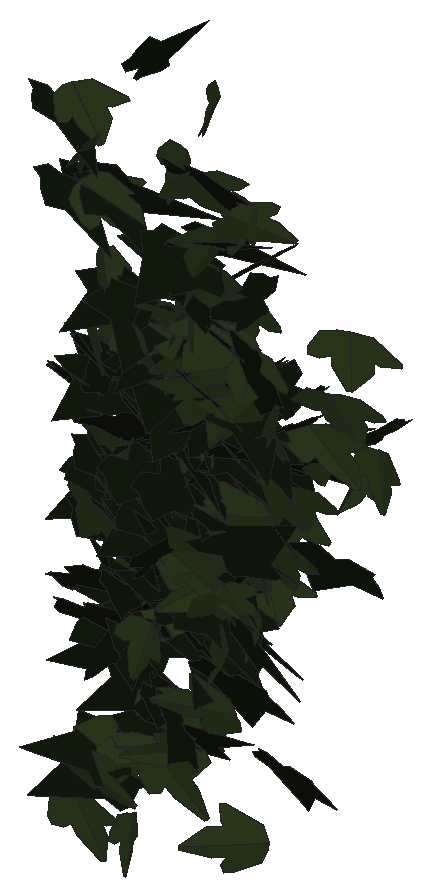
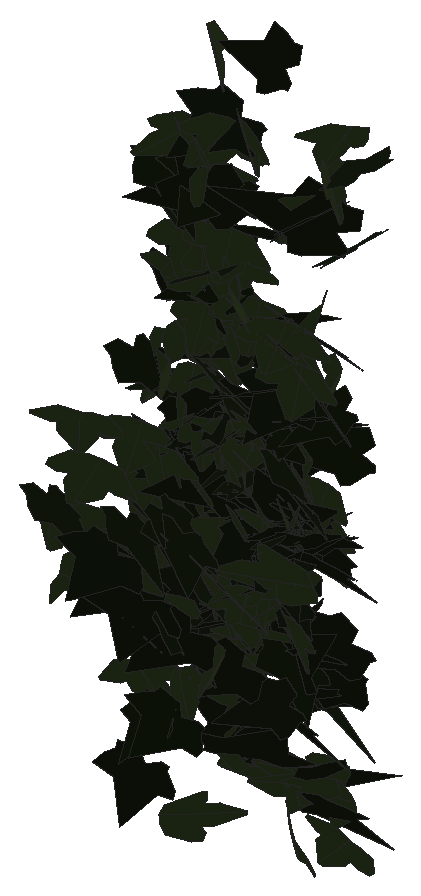
# SketchUp Ruby script. Lengths in millimetres.
U = 1.mm
M = Sketchup.active_model
def pt(a) = Geom::Point3d.new(a.map { |v| v * U })
def face(e, loops, mat)
  f = e.add_face(loops[0].map { |a| pt(a) })
  loops[1..].each { |l| e.add_face(l.map { |a| pt(a) }).erase! }
  f.material = f.back_material = mat if mat
  f
end
# faces: each face lists its corners as indices into pts; further lists are holes
def faces(e, pts, list, mat = nil) = list.each { |f| face(e, (f[0].is_a?(Array) ? f : [f]).map { |l| l.map { |i| pts[i] } }, mat) }
# xy, xz, yz: faces in a plane at the given z, y or x. An outline is a flat list of corners, or four numbers for a rectangle; further outlines are holes
def ring(l) = l.size == 4 ? [[l[0], l[1]], [l[2], l[1]], [l[2], l[3]], [l[0], l[3]]] : l.each_slice(2).to_a
def flat(e, list, mat, &to3) = list.each { |f| face(e, (f[0].is_a?(Array) ? f : [f]).map { |l| ring(l).map { |u, v| to3.(u, v) } }, mat) }
def xy(e, z, list, mat = nil) = flat(e, list, mat) { |x, y| [x, y, z] }
def xz(e, y, list, mat = nil) = flat(e, list, mat) { |x, z| [x, y, z] }
def yz(e, x, list, mat = nil) = flat(e, list, mat) { |y, z| [x, y, z] }
def lines(e, pts, list) = list.each { |a, b| e.add_line(pt(pts[a]), pt(pts[b])) }
# prism: a flat outline (further loops are holes) pulled along v
def prism(e, loops, v, mat = nil)
  f = face(e, loops, mat); d = Geom::Vector3d.new(v.map { |x| x * U })
  f.pushpull(f.normal.samedirection?(d) ? d.length : -d.length)
end
def box(e, o, s, mat = nil) = prism(e, [[o, [o[0] + s[0], o[1], o[2]], [o[0] + s[0], o[1] + s[1], o[2]], [o[0], o[1] + s[1], o[2]]]], [0, 0, s[2]], mat)
def at(x, y, z, deg = 0) = Geom::Transformation.translation(pt([x, y, z])) * Geom::Transformation.rotation(ORIGIN, Z_AXIS, deg.degrees)
def axes(o, x, y, z) = Geom::Transformation.new([*x, 0, *y, 0, *z, 0, *pt(o).to_a, 1])
def part(name) = M.definitions.add(name)
# library, detail: a bought-in or finely detailed component or shape, given as its bounding box
def library(name, o, s) = part(name).tap { |d| box(d.entities, o, s) }
def detail(e, o, s) = box(e.add_group.entities, o, s)
def put(e, d, t, mat = nil) = e.add_instance(d, t).tap { |i| i.material = mat if mat }
def group(e, t, mat = nil) = e.add_group.tap { |g| g.transformation = t; g.material = mat if mat }.entities
root = M.entities
M.materials.add("efeu1").color = [18, 25, 13]
M.materials.add("efeu2").color = [43, 57, 29]
c1 = part("ivyleaf_9")
p = [[39.1,54.8,31.7],[34.5,51.8,30.2],[-5.3,25.2,17.3],[-17.9,28.3,20.9],[-21.6,21.7,17],[-20.2,4.3,5.3],
  [-22.9,-0.3,2.5],[-17.1,-4,-0.6],[-2,-2.1,-1.2],[-0.7,-15.4,-10.1],[16.6,-22.3,-16.7],[21.1,-15.1,-12.5],
  [32.7,-10.7,-11],[46.1,-1.8,-6.6],[30.8,11.2,3.8]]
faces(c1.entities,p,[[0,1,2,3,4,5,6,7,8,9,10,11,12,13,14]],"efeu1")
c2 = part("ivyleaf_10")
p = [[0,12.8,-0.8],[-1.5,51.3,-10.9],[-4.9,51,-11.6],[-13.6,26.5,-7.3],[-13.2,15.9,-4.6],[-21.1,19.3,-7.2],
  [-29.5,16.3,-8.3],[-29.2,8.3,-6.2],[-19.7,-9.8,0.5],[-7.6,-13,4],[1,-12.2,5.8],[-0.4,51.1,-11.1],
  [-1.5,51.1,-10.9],[1,-12.4,5.9],[16.9,-12.4,3.5],[35.1,9.1,-5.1],[35,12.9,-6.1],[20.5,16.4,-4.9],
  [15.8,15,-3.8],[15.3,27.6,-7.1],[12.8,31.3,-7.8]]
faces(c2.entities,p,[[0,1,2,3,4,5,6,7,8,9,10],[11,12,0,13,14,15,16,17,18,19,20]],"efeu2")
put(root,c1,axes([3673.6,933.8,2008.3],[-1.71532,0.04055,0.01997],[-0.04734,-0.11203,-0.89509],[-0.07184,-0.89452,0.11301]))
put(root,c1,axes([3633.8,892.5,2375.7],[0.49599,-0.92629,-0.17661],[-0.02252,0.18,-0.96155],[1.79453,0.25827,0.03674]))
put(root,c1,axes([3632.3,890.9,2463.7],[0.18435,-0.94135,0.27937],[0.2943,-0.26259,-0.93845],[1.84548,0.13591,0.12175]))
put(root,c1,axes([3621.6,907.3,2137],[1.51771,-0.42905,0.25621],[0.48544,-0.06545,-0.9035],[0.81787,0.83504,0.06083]))
put(root,c2,axes([3662.9,917.6,2079.5],[-1.57272,0.45852,0.04383],[-0.08821,0.00679,-0.9449],[-0.87218,-0.82749,0.01653]))
put(root,c1,axes([3685.3,905.5,1840.2],[-1.14241,0.84092,0.03289],[-0.03684,0.02659,-1.03317],[-1.60123,-0.60057,0.00031]))
put(root,c1,axes([3635.1,909.2,1905.6],[1.52663,0.25674,0.39294],[0.70805,0.12662,-0.8422],[-0.54468,0.88419,0.00651]))
put(root,c2,axes([3659.8,1097.4,1962.1],[-0.8183,0.80707,0.14351],[-0.0896,0.13748,-0.91417],[-1.55754,-0.43193,-0.02281]))
put(root,c1,axes([3647.9,912.1,1868.8],[1.7241,0.26652,-0.11191],[-0.20646,-0.02779,-0.94428],[-0.50994,0.91236,0.00393]))
put(root,c1,axes([3642.4,908.2,2180.9],[1.4894,-0.46447,-0.25853],[-0.34559,0.19885,-0.90691],[0.95083,0.79983,0.07534]))
put(root,c1,axes([3686.7,906.5,1696.9],[-1.77573,-0.06272,0.18686],[-0.35243,-0.03072,-0.93496],[0.12848,-0.95105,0.01788]))
put(root,c1,axes([3688.4,1086.8,2056.5],[-1.34517,0.55722,0.10387],[-0.13983,0.07455,-0.89993],[-1.06966,-0.71048,-0.01297]))
put(root,c1,axes([3688.9,901.6,1719.6],[-0.82429,-0.21345,0.80804],[-1.3079,-0.42699,-0.48113],[0.90523,-0.81129,0.04063]))
put(root,c2,axes([3681.3,880.4,2011],[-1.3261,0.43299,0.38568],[-0.75303,0.08574,-0.81106],[-0.80674,-0.79177,0.12309]))
put(root,c2,axes([3661.1,897.6,2214.7],[-0.71641,0.86082,-0.25507],[0.11633,-0.25136,-0.93854],[-1.70476,-0.37891,0.04314]))
put(root,c1,axes([3651.4,930,2047.7],[0.24151,-0.91044,-0.05985],[-0.03003,0.05823,-0.91921],[1.73623,0.12765,-0.00757]))
put(root,c1,axes([3656.9,932.6,2023.4],[-0.24965,-0.9069,0.01351],[0.00625,-0.01413,-0.91633],[1.7262,-0.13111,0.00527]))
put(root,c1,axes([3680.8,942.3,1886.8],[0.11527,0.89691,-0.00348],[0.00089,-0.00352,-0.89895],[-1.70701,0.06057,-0.00071]))
put(root,c2,axes([3673.5,953.1,1932.2],[1.08008,-0.65356,-0.19834],[-0.1506,0.19322,-0.86311],[1.29112,0.56927,0.06525]))
put(root,c1,axes([3671.3,935.7,2031.8],[-0.96682,-0.73449,-0.17827],[0.20746,0.14135,-0.893],[1.42342,-0.51948,0.00907]))
put(root,c2,axes([3652,889.4,1649.2],[1.47018,-0.15436,0.51226],[0.98157,-0.02442,-0.78509],[0.27078,0.92657,0.06465]))
put(root,c2,axes([3680,880.1,2443.5],[0.12874,-0.98974,-0.17322],[-0.00011,0.17361,-0.99198],[1.91231,0.06664,0.01161]))
put(root,c1,axes([3700.6,883.6,2176.2],[-0.37681,0.67605,0.75201],[-0.40511,0.72125,-0.70444],[-1.88143,-0.2907,0.00107]))
put(root,c2,axes([3675.4,943.3,1979.2],[0.6443,0.79194,-0.24251],[-0.28138,-0.19999,-0.85949],[-1.55099,0.36526,0.05519]))
put(root,c2,axes([3666.6,875.2,2492.4],[0.80908,0.86432,0.23318],[0.15964,0.21854,-0.96299],[-1.69629,0.43282,0.02059]))
put(root,c2,axes([3692.5,913.5,2111.1],[0.7486,-0.38137,0.77451],[-1.07561,0.52963,0.54781],[-1.24205,-0.68852,-0.0076]))
put(root,c1,axes([3692.1,908.3,2150.2],[-1.39319,-0.49642,0.31362],[-0.37268,-0.26614,-0.87834],[1.05356,-0.75059,0.10402]))
put(root,c1,axes([3653.6,989.4,1859.6],[1.57955,-0.29876,0.07791],[0.14587,-0.0171,-0.88203],[0.56922,0.83342,0.00983]))
put(root,c1,axes([3701.1,936.6,1868.7],[0.44897,-0.56937,0.88839],[-0.70102,0.80863,0.61605],[-1.88191,-0.43705,-0.01754]))
put(root,c1,axes([3673.8,1143.5,1905.5],[0.93234,0.63225,0.44227],[0.43948,0.37974,-0.79862],[-1.40117,0.5398,0.04379]))
put(root,c2,axes([3678.9,903.4,2290.8],[-0.04781,0.92926,-0.26709],[-0.02416,-0.26748,-0.9294],[-1.84001,-0.02063,0.01914]))
put(root,c2,axes([3660.3,890.3,1702.9],[-0.55459,0.19597,-0.84689],[1.32875,-0.47938,-0.35115],[-0.98562,-0.75653,0.00313]))
put(root,c1,axes([3678.8,946,1845.8],[-0.77992,-0.92763,-0.36512],[0.27358,0.33565,-1.01411],[1.87747,-0.43426,-0.0039]))
put(root,c1,axes([3688.7,941.2,1891],[-1.20376,-0.62089,-0.15637],[0.30026,0.0619,-0.8839],[1.181,-0.64859,0.06534]))
put(root,c2,axes([3689.4,920.3,2060.8],[-0.55356,0.87086,-0.01631],[-0.19104,-0.0506,-0.91139],[-1.64667,-0.28689,0.11122]))
put(root,c2,axes([3697.3,915,2208.3],[-1.77322,0.17086,0.08642],[-0.1535,0.03915,-0.94694],[-0.33051,-0.93488,-0.02386]))
put(root,c1,axes([3712.1,920.9,2097.4],[-0.69109,0.85796,0.0877],[-0.04289,0.08569,-0.93156],[-1.64082,-0.3636,-0.01259]))
put(root,c1,axes([3709.3,905.8,2263.1],[-1.7922,0.09839,-0.16926],[0.27296,-0.21934,-0.92542],[-0.25364,-0.93129,0.20007]))
put(root,c1,axes([3705.4,931.4,1979.3],[-0.19569,0.86544,-0.20515],[0.09309,-0.2007,-0.87119],[-1.69019,-0.11125,-0.02423]))
put(root,c2,axes([3697.7,909.9,2084.3],[0.8017,-0.84181,-0.02418],[-0.01234,0.02379,-0.94131],[1.60275,0.42126,0.00485]))
put(root,c1,axes([3683.5,911.3,1919.9],[0.95433,-0.62284,-0.48454],[-0.53446,0.39567,-0.79921],[1.40353,0.57417,0.02513]))
put(root,c1,axes([3719,919.2,1802.1],[-1.59107,0.31556,-0.01671],[0.0298,-0.00583,-0.89357],[-0.60067,-0.83614,-0.00008]))
put(root,c2,axes([3700.4,1102.4,1922.8],[-0.13731,-0.91445,-0.08181],[0.09265,0.07814,-0.91632],[1.74487,-0.07611,0.04222]))
put(root,c1,axes([3692.5,932.5,2049.3],[-1.24832,0.08888,0.63468],[1.19641,-0.08744,0.6619],[0.23727,0.90851,0.00162]))
put(root,c2,axes([3700.6,915.8,2072.8],[-1.41826,0.5426,-0.01916],[0.03178,-0.00962,-0.92181],[-1.03283,-0.74538,-0.00205]))
put(root,c2,axes([3670.4,895.9,1725.2],[0.28044,0.12175,-1.01603],[1.67002,0.51309,0.18874],[1.00198,-0.88925,-0.03021]))
put(root,c2,axes([3700.4,927.6,2061.9],[0.8884,-0.78576,0.08376],[0.08647,-0.07043,-0.91395],[1.50144,0.46899,0.00308]))
put(root,c1,axes([3684,909.6,1997.7],[1.30839,-0.54835,-0.26594],[-0.33255,0.20672,-0.87793],[1.11119,0.70753,0.0504]))
put(root,c1,axes([3713.6,1086.4,2085.7],[0.28701,0.86465,0.2661],[-0.11277,0.27864,-0.87179],[-1.71807,0.12615,0.10167]))
put(root,c1,axes([3692.4,935.4,2035.8],[-0.25078,-0.86286,-0.26158],[0.03165,0.26199,-0.87258],[1.7157,-0.13095,-0.02214]))
put(root,c2,axes([3707.8,928.1,2062.4],[0.49554,-0.88612,0.04843],[0.03813,-0.04459,-0.92355],[1.68854,0.26105,0.00664]))
put(root,c1,axes([3673.9,934.2,1954.5],[1.20184,-0.53306,0.33993],[0.58025,-0.16414,-0.82376],[1.05409,0.69813,0.06588]))
put(root,c2,axes([3667.5,958.7,1989.3],[0.44823,0.13556,1.03923],[1.80336,0.42759,-0.27051],[-0.8523,0.97603,-0.02583]))
put(root,c1,axes([3690.5,944.4,1953.2],[0.35667,-0.87156,-0.08214],[-0.00877,0.08302,-0.89138],[1.66607,0.18702,0.01289]))
put(root,c2,axes([3704.3,945.6,1962],[-0.67994,-0.81536,-0.11006],[0.4707,0.00801,-0.86217],[1.49345,-0.37374,0.22162]))
put(root,c2,axes([3691.9,869.8,2390],[0.61478,0.79126,0.65933],[0.49777,0.60533,-0.85459],[-1.89596,0.4155,-0.01057]))
put(root,c2,axes([3741.5,879.5,2220.3],[-0.65799,0.15548,0.96307],[-1.72579,0.32558,-0.37808],[-0.68468,-0.97007,0.02747]))
put(root,c1,axes([3685.7,895.9,2004.7],[-0.68785,-0.14762,-0.92172],[1.65761,0.30226,-0.38992],[0.63915,-0.94277,0.01931]))
put(root,c1,axes([3692.2,890.4,2390.5],[0.35411,-0.92804,-0.29168],[-0.01544,0.29547,-0.9453],[1.85137,0.17997,0.04791]))
put(root,c1,axes([3706.3,886.2,2124.4],[1.58719,0.60909,-0.12871],[-0.19721,-0.07635,-1.0327],[-1.16829,0.84037,-0.00053]))
put(root,c1,axes([3708,1135.4,1899.4],[1.34652,-0.15041,-0.56051],[-0.92493,0.3295,-0.70186],[0.60367,0.84034,0.17488]))
put(root,c1,axes([3688.2,920.3,2049.2],[0.84329,-0.86355,0.20883],[0.16488,-0.19025,-0.97055],[1.68283,0.45138,-0.00955]))
put(root,c2,axes([3693,899,1710.6],[0.23826,0.06353,-0.9519],[1.24569,0.69275,0.13232],[1.32097,-0.66474,0.04691]))
put(root,c1,axes([3729.9,1087.7,1979.2],[-0.89479,0.7237,-0.34333],[0.39298,-0.27515,-0.86274],[-1.47296,-0.51304,-0.02161]))
put(root,c1,axes([3671.2,891,2381.4],[1.00697,-0.12814,0.96083],[1.7784,-0.22372,-0.54439],[0.49067,1.07382,0.00124]))
put(root,c1,axes([3697.8,939.4,2030],[0.79982,-0.79543,-0.09642],[0.00516,0.1103,-0.89803],[1.52494,0.41683,0.05362]))
put(root,c2,axes([3705.9,904.7,1640.8],[0.97007,-0.55797,0.59763],[0.73939,-0.45439,-0.75557],[1.36919,0.6407,-0.0154]))
put(root,c1,axes([3703.8,1091.7,1974.6],[1.71986,0.21326,-0.00118],[0.00926,-0.02576,-0.92812],[-0.40578,0.9033,-0.02619]))
put(root,c2,axes([3721.4,910.3,2248.9],[-1.62044,-0.39436,-0.18271],[0.37818,0.0042,-0.93506],[0.73568,-0.8708,0.07823]))
put(root,c2,axes([3720.5,939.2,1911.9],[-0.34348,0.75935,-0.45575],[-0.04259,-0.46888,-0.77236],[-1.68497,-0.14294,0.11243]))
put(root,c1,axes([3740.8,1081.4,2101.7],[-0.80414,0.70772,-0.39931],[0.23909,-0.38777,-0.82018],[-1.52795,-0.43314,0.08181]))
put(root,c1,axes([3718.6,899.4,2176],[1.77263,-0.09802,-0.35514],[-0.67049,0.04552,-0.93651],[0.20514,0.99577,0.00785]))
put(root,c1,axes([3727.5,936.7,2052],[-1.29476,-0.41985,-0.43111],[0.78244,0.15088,-0.79571],[0.83633,-0.79114,0.07703]))
put(root,c2,axes([3724.2,942.7,1898.7],[1.51901,0.41228,0.0331],[0.066,0.00498,-0.89826],[-0.78441,0.79881,-0.01148]))
put(root,c1,axes([3712.3,993.7,1887.9],[1.69486,0.04618,0.03504],[0.06595,0.00842,-0.8917],[-0.08845,0.89118,0.00661]))
put(root,c1,axes([3754.4,937.2,1743.8],[-1.91641,-0.35404,0.19197],[0.36027,0.04022,1.06708],[-0.67654,1.02429,0.02446]))
put(root,c1,axes([3733.7,899.8,2257.4],[-0.97642,-0.81769,0.05598],[-0.00397,-0.06474,-0.96476],[1.55986,-0.51201,0.03259]))
put(root,c1,axes([3744.7,902.6,1999],[-1.11286,-0.44155,0.53269],[-0.39793,-0.55207,-0.68712],[1.25526,-0.56647,0.25443]))
put(root,c2,axes([3726.6,931.8,2024],[1.6998,-0.04927,0.11951],[0.23185,0.04166,-0.8932],[0.0823,0.90012,0.04788]))
put(root,c1,axes([3713.9,902.4,2134.5],[1.37462,-0.61928,-0.08191],[-0.12816,0.0473,-0.95138],[1.18196,0.72536,-0.00789]))
put(root,c1,axes([3721.9,932.2,2013.9],[1.63427,0.27287,0.05516],[0.0478,0.1022,-0.89654],[-0.52768,0.85437,0.08963]))
put(root,c2,axes([3737.5,891,1881.7],[1.33886,-0.63415,0.16529],[0.23437,-0.11025,-0.94712],[1.22502,0.71418,0.00055]))
put(root,c2,axes([3745,940.6,1935.7],[-1.22336,-0.61654,-0.1417],[0.32896,0.02316,-0.88486],[1.15818,-0.65782,0.10165]))
put(root,c2,axes([3751,1109.6,1923.7],[1.2651,0.56842,-0.29043],[-0.66353,-0.02793,-0.85263],[-1.01763,0.72486,0.19489]))
put(root,c1,axes([3733.5,914.6,1803.6],[0.8365,-0.62135,-0.47233],[-0.50457,0.39099,-0.76105],[1.39713,0.51323,0.00795]))
put(root,c2,axes([3770.3,921.6,1741.9],[0.36407,0.23199,-0.85565],[-1.43479,-0.41804,-0.28188],[-0.88784,0.7707,0.10466]))
put(root,c1,axes([3761.2,913,1918.4],[-0.47064,0.19387,0.87259],[-1.13641,-0.70956,-0.01157],[1.26597,-0.56487,0.31401]))
put(root,c1,axes([3766.1,921.8,2086.2],[-1.53532,0.38177,-0.19856],[0.30566,-0.12429,-0.89146],[-0.75981,-0.82143,0.0426]))
put(root,c1,axes([3732.6,877.1,2085.7],[0.36897,-0.58216,-0.75185],[-0.08716,0.76071,-0.60083],[1.80763,0.15551,0.1245]))
put(root,c2,axes([3741.6,936.7,2059.7],[0.94681,-0.62812,0.43089],[0.4963,-0.34311,-0.80123],[1.36209,0.56164,-0.00758]))
put(root,c1,axes([3777.9,1094.6,1961.7],[-1.43218,0.53567,0.06161],[-0.13729,0.00482,-0.92292],[-1.01698,-0.75501,0.03782]))
put(root,c1,axes([3752.6,1104.9,1998.9],[1.02815,0.7173,-0.01855],[-0.01993,-0.01533,-0.89797],[-1.36548,0.54032,-0.00086]))
put(root,c1,axes([3762.5,898.8,1927.6],[0.36282,0.88377,0.03705],[0.013,0.03643,-0.9041],[-1.68342,0.19075,0.001]))
put(root,c1,axes([3774.5,1085.5,2097.9],[-1.46331,0.45023,-0.18621],[0.26691,-0.12864,-0.89013],[-0.88803,-0.78057,0.03929]))
put(root,c2,axes([3746.6,887.9,2235],[1.50407,0.54311,0.12149],[0.07868,0.15313,-0.95348],[-1.05627,0.78477,0.10197]))
put(root,c1,axes([3740.7,884.6,2550],[0.2717,-0.10002,0.98469],[1.33486,0.71219,-0.02934],[-1.3291,0.69483,0.17182]))
put(root,c1,axes([3767.9,897.9,2228.8],[-1.69641,0.05033,-0.37053],[0.64826,-0.2859,-0.85823],[-0.29362,-0.92198,0.24591]))
put(root,c1,axes([3743.4,911.3,2018.1],[-0.32419,-0.89138,-0.29933],[0.23641,0.28021,-0.90511],[1.77388,-0.20025,0.06592]))
put(root,c2,axes([3764.1,900.3,2255.5],[-1.79401,-0.21997,-0.04757],[0.09219,0.00174,-0.96791],[0.41829,-0.94382,0.0093]))
put(root,c2,axes([3748.7,920,1794.9],[1.49096,0.35112,0.25277],[0.42465,0.12006,-0.8583],[-0.70544,0.81436,0.01756]))
put(root,c1,axes([3763.3,891,2202.4],[-1.49486,-0.26057,-0.4574],[0.84512,0.11328,-0.82706],[0.53806,-0.90184,0.02827]))
put(root,c2,axes([3755.4,920.4,1913.1],[1.24575,0.6089,0.12715],[0.20348,0.0717,-0.89375],[-1.16623,0.66292,-0.02012]))
put(root,c1,axes([3783.6,1090.3,2078],[-0.4139,0.8807,-0.01749],[-0.0058,-0.01876,-0.90712],[-1.67647,-0.21737,0.00746]))
put(root,c1,axes([3796.8,885,2227],[-0.28467,0.48576,0.81588],[-0.8958,0.67939,-0.49079],[-1.56951,-0.47587,0.13214]))
put(root,c2,axes([3736.9,918.9,2025.3],[0.81719,-0.03804,0.80607],[1.40734,0.38414,-0.37576],[-0.61494,0.82859,0.21121]))
put(root,c1,axes([3758,939.5,1932.8],[-0.24414,-0.89547,-0.05421],[0.00359,0.0545,-0.90459],[1.70737,-0.12816,-0.00585]))
put(root,c1,axes([3756.5,910.8,1949.4],[1.30625,-0.3354,-0.48287],[-0.59331,0.4217,-0.73601],[0.94869,0.72554,0.20457]))
put(root,c1,axes([3786.2,1051,1965.1],[-0.10233,0.84026,0.33725],[-0.17075,0.33124,-0.83959],[-1.71471,-0.08313,0.06348]))
put(root,c2,axes([3761.1,915.5,2094.1],[1.32915,0.56841,0.20975],[0.07453,0.27705,-0.8812],[-1.15069,0.67451,0.1852]))
put(root,c1,axes([3794,885.6,2130.2],[-0.64083,0.86964,0.09789],[-0.19701,0.06457,-0.9297],[-1.65386,-0.34466,0.07282]))
put(root,c1,axes([3753.9,875.7,1974.5],[0.5051,0.09517,0.92197],[1.30019,0.62804,-0.26148],[-1.19216,0.72527,0.10545]))
put(root,c1,axes([3751.6,924.7,2074.1],[1.0617,-0.69879,-0.16171],[-0.05375,0.1833,-0.88952],[1.36402,0.55113,0.09081]))
put(root,c2,axes([3778,927.7,2019.7],[0.96539,-0.73779,-0.19012],[-0.1422,0.17914,-0.89449],[1.44305,0.51123,0.03905]))
put(root,c2,axes([3744.3,912.3,1721.8],[1.08882,-0.09006,0.82312],[1.54758,-0.12771,-0.57915],[0.29741,0.99424,0.00016]))
put(root,c1,axes([3779.3,907.2,2153.9],[-1.00859,-0.75342,0.2715],[-0.00929,-0.32251,-0.90452],[1.52414,-0.50054,0.17415]))
put(root,c2,axes([3782.1,907,2269.6],[0.53753,-0.82574,0.40425],[0.21901,-0.38782,-0.87257],[1.73601,0.30461,-0.01509]))
put(root,c2,axes([3786.8,911.9,2123.9],[1.41764,-0.56647,-0.14982],[-0.1951,0.1126,-0.9354],[1.09798,0.7514,0.02723]))
put(root,c2,axes([3783.8,902.8,2225.2],[-0.20971,-0.75305,0.59379],[0.31368,-0.60367,-0.735],[1.798,0.01749,0.19748]))
put(root,c2,axes([3800.4,934.3,1966.3],[-1.5352,0.27027,0.33586],[-0.66482,0.00779,-0.84524],[-0.4808,-0.87373,0.09635]))
put(root,c2,axes([3781.9,939.4,2010.1],[1.08462,0.70089,-0.06359],[-0.20822,0.0074,-0.89891],[-1.32313,0.57338,0.08934]))
put(root,c2,axes([3787.2,1095.8,2027.8],[-1.71786,-0.00996,-0.06789],[0.129,0.00991,-0.90263],[0.02031,-0.90511,-0.00914]))
put(root,c1,axes([3752.2,918.3,1761.3],[1.45129,0.26444,-0.41131],[0.74175,0.1315,0.8071],[0.56204,-0.85637,-0.00308]))
put(root,c2,axes([3787.3,902.7,1985.4],[1.22649,-0.57343,-0.28787],[-0.03036,0.39356,-0.81966],[1.22077,0.5859,0.26884]))
put(root,c1,axes([3779.9,902.3,1778],[-0.1498,-0.49549,0.82496],[-0.28871,-0.81097,-0.50157],[1.8086,-0.1705,-0.01174]))
put(root,c1,axes([3796.4,892.2,2342.5],[-1.55127,-0.53147,0.11797],[0.0792,-0.27261,-0.94058],[1.03309,-0.77715,0.24926]))
put(root,c2,axes([3787.9,907.7,2115.1],[0.24655,0.80433,0.45266],[-0.30966,0.46984,-0.7883],[-1.72907,0.03055,0.20572]))
put(root,c1,axes([3768.5,913.3,1900.8],[1.24811,-0.65148,-0.14998],[-0.20357,0.10514,-0.92438],[1.25593,0.66446,-0.00079]))
put(root,c1,axes([3772.7,1088.1,2014.5],[1.49788,0.45811,0.21935],[0.36171,0.10952,-0.91065],[-0.89643,0.80965,-0.00093]))
put(root,c1,axes([3776,874.8,2085.6],[0.40613,-0.50269,-0.82813],[-0.25942,0.82397,-0.53529],[1.82541,0.22894,0.10818]))
put(root,c1,axes([3814.4,929.1,1925.4],[-0.85502,0.78437,0.09153],[-0.07017,0.08436,-0.90386],[-1.50129,-0.45066,-0.00988]))
put(root,c2,axes([3789.9,883.4,2457],[1.17122,-0.78959,0.04184],[0.17391,0.01836,-0.99762],[1.49478,0.61654,0.08328]))
put(root,c2,axes([3787.3,921.9,2074.3],[1.061,-0.7265,0.19251],[0.32738,-0.10998,-0.91322],[1.39243,0.57944,0.06803]))
put(root,c1,axes([3774.3,906.5,2113.4],[0.55936,-0.86361,0.2712],[0.11433,-0.2659,-0.91183],[1.71896,0.29871,-0.0276]))
put(root,c1,axes([3811.4,909.2,2141],[-0.16796,0.67183,-0.67181],[0.07028,-0.67176,-0.67664],[-1.80685,-0.08858,0.03613]))
put(root,c2,axes([3803.5,899.5,2328.8],[-1.8468,0.08047,0.01787],[-0.03412,0.00006,-0.9737],[-0.15313,-0.97053,0.00142]))
put(root,c1,axes([3790.2,1103.7,2041.9],[1.11579,0.6395,0.26381],[0.33937,0.19442,-0.86757],[-1.27211,0.61279,-0.00006]))
put(root,c2,axes([3811,893.8,2298.9],[-1.75425,-0.29114,0.09967],[-0.13788,-0.10058,-0.96381],[0.56921,-0.92164,0.0737]))
put(root,c1,axes([3782.9,919.8,1979.8],[0.65291,-0.83725,-0.24043],[0.01899,0.26216,-0.89869],[1.65774,0.32675,0.10499]))
put(root,c1,axes([3831.4,888.9,2154.3],[-1.12452,0.70866,0.1372],[-0.228,0.07857,-0.92175],[-1.35472,-0.60147,0.04125]))
put(root,c2,axes([3818.7,894.1,1963.1],[0.65598,0.38691,-0.74989],[-0.99917,-0.53585,-0.51777],[-1.2573,0.6277,0.02022]))
put(root,c1,axes([3789.1,920.2,2100.4],[0.23858,-0.87706,0.22262],[0.04294,-0.22165,-0.88593],[1.72163,0.12707,-0.00875]))
put(root,c2,axes([3810.7,929,2115.2],[-0.72243,-0.81563,-0.17559],[0.13392,0.16093,-0.89963],[1.58222,-0.38603,-0.00403]))
put(root,c1,axes([3786.9,925.3,2106.5],[0.70761,-0.83673,-0.16505],[0.01907,0.18433,-0.91188],[1.62305,0.36263,0.08267]))
put(root,c1,axes([3782.8,920.3,2048.3],[1.20571,0.26515,0.61168],[1.03133,0.28673,-0.68553],[-0.73911,0.83264,0.04128]))
put(root,c2,axes([3842.8,883.4,1830.9],[-0.51301,0.05015,0.89638],[-1.65592,-0.24532,-0.24792],[0.42124,-0.90331,0.11709]))
put(root,c1,axes([3790.4,918.1,2069.9],[0.83022,-0.82316,-0.10756],[-0.09587,0.09504,-0.9316],[1.57705,0.43912,-0.00001]))
put(root,c2,axes([3823.3,884.8,2198.3],[-1.42601,-0.55932,0.22375],[-0.29686,-0.16479,-0.93425],[1.10742,-0.7644,0.03769]))
put(root,c2,axes([3799.4,889.1,2294],[0.50106,-0.71145,0.6138],[0.85689,-0.46398,-0.73091],[1.56964,0.4804,0.20308]))
put(root,c2,axes([3829.7,945.9,1645.3],[-0.3204,0.13796,1.07578],[-0.53994,-1.05636,0.09107],[1.99233,-0.2641,0.19768]))
put(root,c2,axes([3807.1,927.7,2117.3],[1.05738,0.72457,0.05902],[0.08953,0.03829,-0.91295],[-1.38067,0.55739,-0.014]))
put(root,c1,axes([3816,920.4,2078],[-1.01955,-0.73522,-0.04467],[0.13611,0.00305,-0.90797],[1.39523,-0.53755,0.05594]))
put(root,c1,axes([3796.3,884.8,2308.3],[1.31422,-0.57375,-0.43415],[-0.26809,0.4823,-0.86143],[1.34285,0.65781,0.25292]))
put(root,c2,axes([3816.1,877.6,2225.3],[-1.58587,-0.3656,-0.27601],[0.49069,0.09928,-0.90986],[0.72065,-0.87215,0.01213]))
put(root,c1,axes([3820.4,923.8,1869],[-0.99296,-0.73579,0.27179],[-0.05094,-0.30953,-0.88934],[1.49196,-0.50026,0.15052]))
put(root,c1,axes([3797.8,878.1,2208.7],[1.63675,-0.39274,-0.06197],[-0.09669,0.03793,-0.94534],[0.75051,0.86139,0.01337]))
put(root,c1,axes([3812.6,915.7,2124.8],[1.54595,-0.27945,-0.33574],[-0.57604,0.15106,-0.85802],[0.59944,0.86586,0.04134]))
put(root,c2,axes([3834.7,884.5,2382.7],[-0.65708,-0.90146,0.24674],[-0.05705,-0.25222,-0.96343],[1.77785,-0.34126,0.06028]))
put(root,c2,axes([3834.6,889.1,2264.2],[-1.69928,-0.33818,0.05586],[-0.05989,-0.07432,-0.95297],[0.64959,-0.89151,0.05826]))
put(root,c2,axes([3816.3,988.6,1930.1],[1.43167,0.46618,0.1884],[0.26904,0.12927,-0.88431],[-0.91835,0.76463,0.03464]))
put(root,c2,axes([3819.4,879.2,2442.7],[-1.33522,-0.464,-0.53052],[0.8207,0.3095,-0.84095],[1.06101,-0.82332,-0.01715]))
put(root,c1,axes([3828.3,912,1852.7],[0.62276,0.45031,0.71547],[0.31402,0.71842,-0.52763],[-1.578,0.32068,0.17737]))
put(root,c2,axes([3797.3,882.1,1985.3],[1.09182,-0.03964,0.78885],[1.49147,0.15028,-0.56236],[-0.18767,0.96374,0.12013]))
put(root,c1,axes([3816.7,920.1,2124.3],[0.53698,-0.73153,-0.50728],[-0.35048,0.47268,-0.78405],[1.65759,0.33692,-0.00145]))
put(root,c2,axes([3835,907.1,2232],[-1.39084,0.6038,0.11548],[-0.2372,0.03014,-0.94632],[-1.14569,-0.73924,0.05574]))
put(root,c1,axes([3842.2,917.7,2128.2],[-0.29784,0.49308,-0.76149],[0.27575,-0.74923,-0.51492],[-1.7044,-0.20738,0.04976]))
put(root,c1,axes([3805,886.5,2274.5],[1.70058,-0.43294,0.04999],[0.08023,-0.02765,-0.99288],[0.82556,0.89451,-0.00649]))
put(root,c2,axes([3832.1,932.1,2048],[1.24947,-0.63349,0.00392],[0.00095,-0.00513,-0.91231],[1.20567,0.6565,-0.00334]))
put(root,c1,axes([3799.8,919.4,2017.3],[1.35485,-0.4311,0.38388],[0.69272,-0.13784,-0.82976],[0.85269,0.79696,0.06414]))
put(root,c2,axes([3818.3,886.5,2005.9],[-1.29407,-0.4683,0.53221],[0.82975,0.30527,0.8256],[-1.0639,0.8077,-0.00346]))
put(root,c2,axes([3845.3,880.4,1904.4],[0.43026,-0.76514,-0.70773],[-0.36742,0.68091,-0.79781],[1.94931,0.29723,0.00584]))
put(root,c1,axes([3814.7,868.7,2456.6],[1.91942,-0.06202,-0.08568],[-0.16117,0.01875,-1.01034],[0.12063,1.01198,0.01347]))
put(root,c1,axes([3830,870.2,2379.3],[1.38506,0.63648,0.2004],[-0.01785,0.30626,-0.93863],[-1.26986,0.68992,0.23178]))
put(root,c2,axes([3840.4,874.6,2545.9],[0.53566,-0.94142,-0.25988],[-0.00354,0.26994,-0.97987],[1.85871,0.27182,0.07303]))
put(root,c1,axes([3818.9,933.1,1971.8],[0.408,-0.87178,0.1773],[0.01642,-0.18033,-0.89711],[1.69306,0.21183,-0.03402]))
put(root,c2,axes([3844,883.5,2272.7],[1.63408,0.38619,-0.3853],[-0.69928,-0.1217,-0.94074],[-0.76745,0.93319,0.03677]))
put(root,c2,axes([3839.4,910.3,2154.6],[-0.60878,-0.85172,-0.44466],[0.28868,0.41801,-0.9098],[1.80568,-0.35399,-0.00446]))
put(root,c2,axes([3837.7,931.6,1984.1],[-1.06094,-0.6346,-0.35867],[0.47989,0.25578,-0.84445],[1.30168,-0.61153,0.01899]))
put(root,c2,axes([3816.5,1075.4,2056.3],[1.35631,0.1701,0.58473],[1.07793,0.14557,-0.73262],[-0.42583,0.91027,0.0079]))
put(root,c2,axes([3874.9,899.1,2063.9],[-0.5909,-0.06045,0.86319],[-1.44983,-0.41586,-0.30313],[0.78108,-0.81765,0.09036]))
put(root,c1,axes([3829.6,904.7,1938.4],[-0.50531,-0.78685,-0.50479],[0.46306,0.44851,-0.82709],[1.7179,-0.35234,0.07446]))
put(root,c2,axes([3847.7,1118.5,2006.9],[0.10427,0.54628,-0.75963],[-0.44873,-0.72832,-0.54077],[-1.72328,0.2227,0.09485]))
put(root,c1,axes([3813.6,887.4,2373.2],[1.51644,0.12443,0.54979],[1.03591,0.07771,-0.80642],[-0.27897,0.96493,-0.00595]))
put(root,c1,axes([3845.2,986.8,1719.2],[1.49854,0.04929,-0.48881],[-0.93313,0.02011,-0.78774],[-0.05947,0.92655,0.04311]))
put(root,c2,axes([3846.3,1069.1,2112.1],[-1.72118,-0.12101,-0.21653],[0.41293,0.01089,-0.91225],[0.22883,-0.92986,0.01749]))
put(root,c1,axes([3853.1,940.6,2000.7],[-0.71583,0.37539,-0.96435],[1.05386,-0.79381,-0.52497],[-1.66383,-0.6643,0.08237]))
put(root,c2,axes([3863.8,940.5,2063.5],[-1.64707,0.13442,0.26468],[-0.51075,-0.00554,-0.87466],[-0.24151,-0.90497,0.04467]))
put(root,c2,axes([3856.8,895.9,2309.1],[-1.81705,0.1922,0.0086],[-0.04954,-0.08591,-0.96978],[-0.36279,-0.9509,0.08935]))
put(root,c1,axes([3829.1,916.5,1923.6],[1.67321,-0.33856,-0.02252],[-0.04276,0.00433,-0.94208],[0.64435,0.87943,-0.00403]))
put(root,c2,axes([3844.7,879.9,1966.8],[-0.92934,-0.5347,-0.62054],[0.7804,0.46583,-0.72406],[1.34957,-0.63758,-0.00862]))
put(root,c2,axes([3850.9,931.2,1992.9],[-0.69032,0.84209,-0.06263],[-0.01602,-0.07177,-0.91618],[-1.60702,-0.36102,0.03604]))
put(root,c2,axes([3866.1,891,2190.4],[-0.69514,-0.76946,0.49291],[-0.15054,-0.50221,-0.84259],[1.73261,-0.35235,0.12455]))
put(root,c2,axes([3853,1082.5,2176.3],[1.59341,0.40918,0.04116],[0.06937,0.01915,-0.93187],[-0.77961,0.83802,0.0012]))
put(root,c2,axes([3869.4,900.3,1931.9],[0.87244,-0.82523,-0.32812],[-0.26233,0.29867,-0.94372],[1.66969,0.47812,0.02318]))
put(root,c1,axes([3885.1,1095.3,2075.2],[-0.53687,0.86545,-0.09653],[-0.13497,-0.12396,-0.90415],[-1.65183,-0.27115,0.10525]))
put(root,c1,axes([3864.9,873.7,1881.4],[1.71648,0.14899,-0.53833],[-1.01375,-0.07835,-0.91408],[-0.32,1.04741,0.0082]))
put(root,c1,axes([3902.6,870.9,2254.9],[0.03446,0.13265,-1.05903],[-2.03129,0.00589,-0.01751],[0.00698,1.05917,0.13273]))
put(root,c1,axes([3848.7,883.3,2016.7],[-0.67955,0.16504,0.90378],[1.57554,-0.36269,0.39329],[0.75826,0.90153,-0.00723]))
put(root,c1,axes([3898.5,879.6,2331.9],[-1.16544,0.77049,-0.02027],[0.02237,-0.01655,-0.98419],[-1.46674,-0.61247,0.00109]))
put(root,c2,axes([3872.8,884.3,2424.1],[1.26393,-0.72675,0.02418],[0.10647,0.01841,-0.98301],[1.37981,0.66429,0.0537]))
put(root,c1,axes([3861.5,904.8,2178.5],[-0.14934,-0.95567,0.04922],[0.18242,-0.05699,-0.95365],[1.81209,-0.07302,0.10006]))
put(root,c2,axes([3877.7,928.9,2013.4],[-1.71785,0.17243,-0.09131],[0.1758,-0.00303,-0.91882],[-0.32709,-0.90721,-0.01429]))
put(root,c2,axes([3876.3,920.1,2156.3],[-0.99801,0.7715,-0.06941],[0.08074,-0.05509,-0.93283],[-1.47203,-0.52608,-0.0041]))
put(root,c1,axes([3863,918.3,2145],[-0.04269,-0.89944,0.19745],[0.57938,-0.19365,-0.84753],[1.65403,0.04462,0.30197]))
put(root,c1,axes([3901.3,883.7,2378.9],[-0.20463,0.97207,-0.1177],[0.03599,-0.11632,-0.97798],[-1.8632,-0.109,-0.00596]))
put(root,c2,axes([3881.1,882,2255.1],[1.80551,-0.22191,0.05992],[0.11333,-0.0085,-0.97426],[0.42253,0.95052,0.00527]))
put(root,c1,axes([3905.8,924.2,2169.1],[-0.43869,0.8001,-0.41493],[-0.02026,-0.43067,-0.82454],[-1.71522,-0.19955,0.11586]))
put(root,c2,axes([3894.4,936.2,2081.1],[-1.71436,-0.15961,-0.07893],[0.14514,0.022,-0.91477],[0.30623,-0.90396,-0.00832]))
put(root,c2,axes([3876.7,874,2423],[-0.81473,-0.40328,-0.79271],[1.10006,0.5425,-0.58812],[1.28651,-0.71926,0.00088]))
put(root,c2,axes([3887.3,914.7,2176.7],[0.50866,-0.84253,0.30621],[0.47689,-0.23658,-0.86965],[1.63811,0.33049,0.15809]))
put(root,c2,axes([3881.3,1091.2,2044.1],[1.33117,-0.48932,0.40341],[0.70146,-0.17509,-0.85141],[0.9822,0.78822,0.06131]))
put(root,c1,axes([3878,873.6,1941.3],[1.29337,-0.63242,-0.33134],[-0.42474,0.24635,-0.92794],[1.29072,0.71478,0.02666]))
put(root,c1,axes([3907.6,987.8,1985],[1.09317,0.30633,-0.64526],[-1.09629,-0.29097,-0.65089],[-0.80386,0.8134,0.01017]))
put(root,c1,axes([3876,925.3,2047.3],[0.35693,-0.58114,0.69296],[0.34838,-0.66866,-0.61031],[1.68561,0.26125,-0.0206]))
